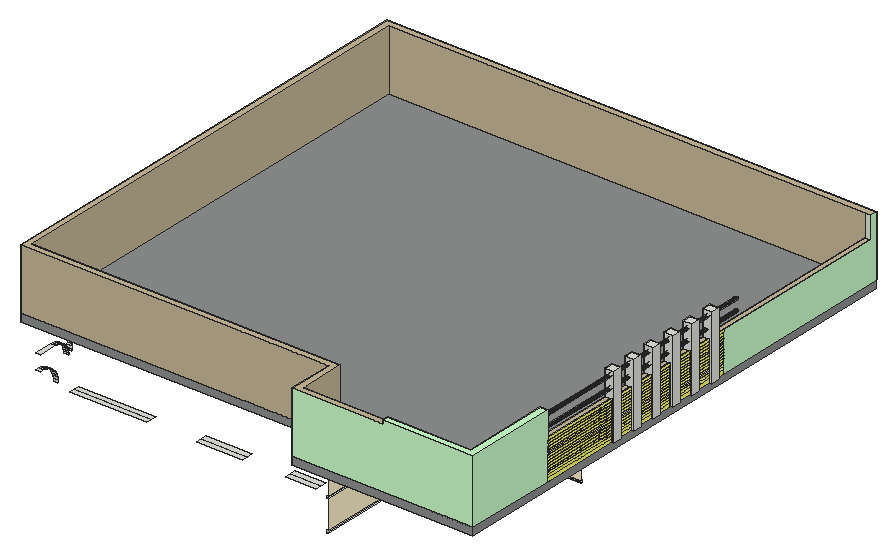
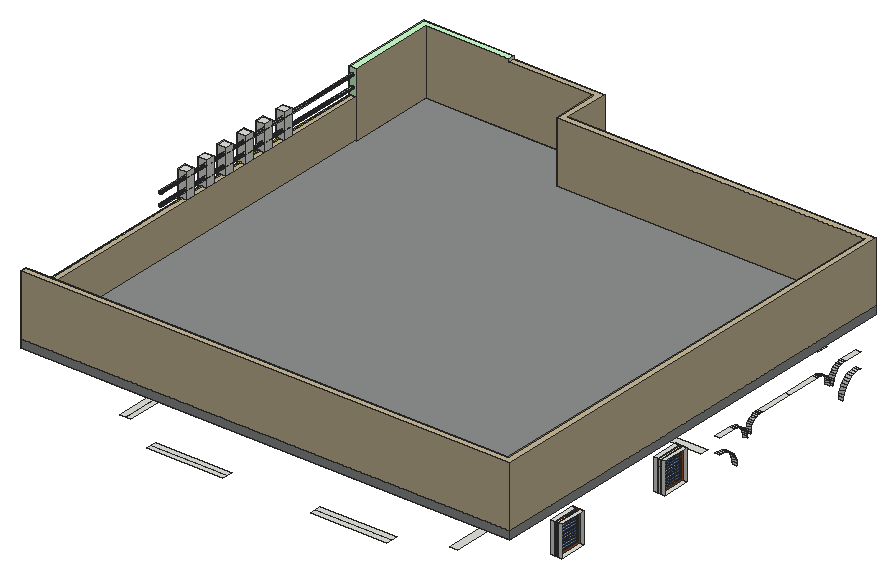
# SketchUp Ruby script. Lengths in inches.
U = 1.inch
M = Sketchup.active_model
def pt(a) = Geom::Point3d.new(a.map { |v| v * U })
def face(e, loops, mat)
  f = e.add_face(loops[0].map { |a| pt(a) })
  loops[1..].each { |l| e.add_face(l.map { |a| pt(a) }).erase! }
  f.material = f.back_material = mat if mat
  f
end
# faces: each face lists its corners as indices into pts; further lists are holes
def faces(e, pts, list, mat = nil) = list.each { |f| face(e, (f[0].is_a?(Array) ? f : [f]).map { |l| l.map { |i| pts[i] } }, mat) }
# xy, xz, yz: faces in a plane at the given z, y or x. An outline is a flat list of corners, or four numbers for a rectangle; further outlines are holes
def ring(l) = l.size == 4 ? [[l[0], l[1]], [l[2], l[1]], [l[2], l[3]], [l[0], l[3]]] : l.each_slice(2).to_a
def flat(e, list, mat, &to3) = list.each { |f| face(e, (f[0].is_a?(Array) ? f : [f]).map { |l| ring(l).map { |u, v| to3.(u, v) } }, mat) }
def xy(e, z, list, mat = nil) = flat(e, list, mat) { |x, y| [x, y, z] }
def xz(e, y, list, mat = nil) = flat(e, list, mat) { |x, z| [x, y, z] }
def yz(e, x, list, mat = nil) = flat(e, list, mat) { |y, z| [x, y, z] }
def lines(e, pts, list) = list.each { |a, b| e.add_line(pt(pts[a]), pt(pts[b])) }
# prism: a flat outline (further loops are holes) pulled along v
def prism(e, loops, v, mat = nil)
  f = face(e, loops, mat); d = Geom::Vector3d.new(v.map { |x| x * U })
  f.pushpull(f.normal.samedirection?(d) ? d.length : -d.length)
end
def box(e, o, s, mat = nil) = prism(e, [[o, [o[0] + s[0], o[1], o[2]], [o[0] + s[0], o[1] + s[1], o[2]], [o[0], o[1] + s[1], o[2]]]], [0, 0, s[2]], mat)
def at(x, y, z, deg = 0) = Geom::Transformation.translation(pt([x, y, z])) * Geom::Transformation.rotation(ORIGIN, Z_AXIS, deg.degrees)
def axes(o, x, y, z) = Geom::Transformation.new([*x, 0, *y, 0, *z, 0, *pt(o).to_a, 1])
def part(name) = M.definitions.add(name)
# library, detail: a bought-in or finely detailed component or shape, given as its bounding box
def library(name, o, s) = part(name).tap { |d| box(d.entities, o, s) }
def detail(e, o, s) = box(e.add_group.entities, o, s)
def put(e, d, t, mat = nil) = e.add_instance(d, t).tap { |i| i.material = mat if mat }
def group(e, t, mat = nil) = e.add_group.tap { |g| g.transformation = t; g.material = mat if mat }.entities
root = M.entities
M.materials.add("[Blacktop Old 02]").color = [143, 145, 145]
M.materials.add("[Color D01]").color = [255, 242, 204]
M.materials.add("[Color E03]").color = [255, 255, 101]
M.materials.add("[Color G01]").color = [204, 255, 204]
M.materials.add("[Metal Aluminum Anodized]").color = [202, 209, 219]
M.materials.add("[Quartz Light Brown]").color = [199, 184, 152]
M.materials.add("[Translucent Glass Blue]").color = [100, 149, 237]
M.materials["[Translucent Glass Blue]"].alpha = 0.5
M.materials.add("[Wood Cherry Original]").color = [152, 86, 42]
c1 = part("Group50\#1")
prism(c1.entities,[[[-9.82,-10.3125,0],[-9.82,-10.89,1],[-9.82,-9.89,1],[-9.82,-9.3125,0]]],[19.64,0,0])
c2 = part("Group51\#1")
prism(c2.entities,[[[-9.82,-7.89,1],[-9.82,-7.3125,0],[-9.82,-8.3125,0],[-9.82,-8.89,1]]],[19.64,0,0])
c3 = part("Group52\#1")
prism(c3.entities,[[[-9.82,-6.3125,0],[-9.82,-6.89,1],[-9.82,-5.89,1],[-9.82,-5.3125,0]]],[19.64,0,0])
c4 = part("Group53\#1")
prism(c4.entities,[[[9.82,-4.89,1],[9.82,-4.3125,0],[9.82,-3.3125,0],[9.82,-3.89,1]]],[-19.64,0,0])
c5 = part("Group54\#1")
prism(c5.entities,[[[-9.82,-1.89,1],[-9.82,-1.3125,0],[-9.82,-2.3125,0],[-9.82,-2.89,1]]],[19.64,0,0])
c6 = part("Group55\#1")
prism(c6.entities,[[[9.82,-0.3125,0],[9.82,0.6875,0],[9.82,0.11,1],[9.82,-0.89,1]]],[-19.64,0,0])
c7 = part("Group56\#1")
prism(c7.entities,[[[-9.82,2.11,1],[-9.82,2.6875,0],[-9.82,1.6875,0],[-9.82,1.11,1]]],[19.64,0,0])
c8 = part("Group57\#1")
prism(c8.entities,[[[-9.82,3.6875,0],[-9.82,3.11,1],[-9.82,4.11,1],[-9.82,4.6875,0]]],[19.64,0,0])
c9 = part("Group58\#1")
prism(c9.entities,[[[9.82,5.11,1],[9.82,5.6875,0],[9.82,6.6875,0],[9.82,6.11,1]]],[-19.64,0,0])
c10 = part("Group59\#1")
prism(c10.entities,[[[9.82,7.11,1],[9.82,7.6875,0],[9.82,8.6875,0],[9.82,8.11,1]]],[-19.64,0,0])
c11 = part("Group60\#1")
prism(c11.entities,[[[-9.82,9.6875,0],[-9.82,9.11,1],[-9.82,10.11,1],[-9.82,10.6875,0]]],[19.64,0,0])
c12 = part("Group48\#1")
put(c12.entities,c1,at(0,0,0),"[Translucent Glass Blue]")
put(c12.entities,c2,at(0,0,0),"[Translucent Glass Blue]")
put(c12.entities,c3,at(0,0,0),"[Translucent Glass Blue]")
put(c12.entities,c4,at(0,0,0),"[Translucent Glass Blue]")
put(c12.entities,c5,at(0,0,0),"[Translucent Glass Blue]")
put(c12.entities,c6,at(0,0,0),"[Translucent Glass Blue]")
put(c12.entities,c7,at(0,0,0),"[Translucent Glass Blue]")
put(c12.entities,c8,at(0,0,0),"[Translucent Glass Blue]")
put(c12.entities,c9,at(0,0,0),"[Translucent Glass Blue]")
put(c12.entities,c10,at(0,0,0),"[Translucent Glass Blue]")
put(c12.entities,c11,at(0,0,0),"[Translucent Glass Blue]")
c13 = part("Group62\#1")
prism(c13.entities,[[[9.56,-10.72,1],[9.56,-10.15,0],[9.56,-9.15,0],[9.56,-9.72,1]]],[-19.11,0,0])
c14 = part("Group63\#1")
prism(c14.entities,[[[-9.56,-7.15,0],[-9.56,-8.15,0],[-9.56,-8.72,1],[-9.56,-7.72,1]]],[19.11,0,0])
c15 = part("Group64\#1")
prism(c15.entities,[[[-9.56,-6.72,1],[-9.56,-5.72,1],[-9.56,-5.15,0],[-9.56,-6.15,0]]],[19.11,0,0])
c16 = part("Group65\#1")
prism(c16.entities,[[[9.56,-4.72,1],[9.56,-4.15,0],[9.56,-3.15,0],[9.56,-3.72,1]]],[-19.11,0,0])
c17 = part("Group66\#1")
prism(c17.entities,[[[-9.56,-2.72,1],[-9.56,-1.72,1],[-9.56,-1.15,0],[-9.56,-2.15,0]]],[19.11,0,0])
c18 = part("Group67\#1")
prism(c18.entities,[[[-9.56,-0.15,0],[-9.56,-0.72,1],[-9.56,0.28,1],[-9.56,0.85,0]]],[19.11,0,0])
c19 = part("Group68\#1")
prism(c19.entities,[[[-9.56,1.85,0],[-9.56,1.28,1],[-9.56,2.28,1],[-9.56,2.85,0]]],[19.11,0,0])
c20 = part("Group69\#1")
prism(c20.entities,[[[9.56,3.85,0],[9.56,4.85,0],[9.56,4.28,1],[9.56,3.28,1]]],[-19.11,0,0])
c21 = part("Group70\#1")
prism(c21.entities,[[[9.56,5.28,1],[9.56,5.85,0],[9.56,6.85,0],[9.56,6.28,1]]],[-19.11,0,0])
c22 = part("Group71\#1")
prism(c22.entities,[[[-9.56,8.85,0],[-9.56,7.85,0],[-9.56,7.28,1],[-9.56,8.28,1]]],[19.11,0,0])
c23 = part("Group72\#1")
xy(c23.entities,0,[[-9.56,9.85,9.56,10.72]])
xy(c23.entities,1,[[-9.56,9.28,9.56,10.28]])
p = [[9.56,9.28,1],[-9.56,9.28,1],[-9.56,9.85,0],[9.56,9.85,0],[-9.56,10.28,1],[9.56,10.28,1],
  [9.56,10.72,0.22],[-9.56,10.72,0.22]]
faces(c23.entities,p,[[0,1,2,3],[4,5,6,7]])
c24 = part("Group60\#2")
put(c24.entities,c13,at(0,0,0))
put(c24.entities,c14,at(0,0,0))
put(c24.entities,c15,at(0,0,0))
put(c24.entities,c16,at(0,0,0))
put(c24.entities,c17,at(0,0,0))
put(c24.entities,c18,at(0,0,0))
put(c24.entities,c19,at(0,0,0))
put(c24.entities,c20,at(0,0,0))
put(c24.entities,c21,at(0,0,0))
put(c24.entities,c22,at(0,0,0))
put(c24.entities,c23,at(0,0,0))
c25 = part("Group234\#2")
xy(c25.entities,126,[[595.96,-36,595.96,0,353.96,0,353.96,360,737.96,360,737.96,355,358.96,355,358.96,5,600.96,5,600.96,-31,666.96,-31,666.96,-36],[666.96,-36,732.27,-31],[732.27,-36,737.96,37.1875],[732.96,37.1875,737.96,355]])
xy(c25.entities,128.53,[[736.96,37.1875,737.96,210.375]])
xy(c25.entities,130.47,[[736.96,37.1875,737.96,210.375]])
xy(c25.entities,130.53,[[736.96,37.1875,737.96,210.375]])
xy(c25.entities,132.47,[[736.96,37.1875,737.96,210.375]])
xy(c25.entities,132.53,[[736.96,37.1875,737.96,210.375]])
xy(c25.entities,134.47,[[736.96,37.1875,737.96,210.375]])
xy(c25.entities,134.53,[[736.96,37.1875,737.96,210.375]])
xy(c25.entities,136.47,[[736.96,37.1875,737.96,210.375]])
xy(c25.entities,136.53,[[736.96,37.1875,737.96,210.375]])
xy(c25.entities,138.47,[[736.96,37.1875,737.96,210.375]])
xy(c25.entities,138.53,[[736.96,37.1875,737.96,210.375]])
xy(c25.entities,140.47,[[736.96,37.1875,737.96,210.375]])
xy(c25.entities,140.53,[[736.96,37.1875,737.96,210.375]])
xy(c25.entities,142.47,[[736.96,37.1875,737.96,210.375]])
xy(c25.entities,142.53,[[736.96,37.1875,737.96,210.375]])
xy(c25.entities,144.47,[[736.96,37.1875,737.96,210.375]])
xy(c25.entities,144.53,[[736.96,37.1875,737.96,210.375]])
xy(c25.entities,146.47,[[736.96,37.1875,737.96,210.375]])
xy(c25.entities,146.53,[[736.96,37.1875,737.96,210.375]])
xy(c25.entities,148.47,[[736.96,37.1875,737.96,210.375]])
xy(c25.entities,148.53,[[736.96,37.1875,737.96,210.375]])
xy(c25.entities,150.47,[[736.96,37.1875,737.96,210.375]])
xy(c25.entities,150.53,[[736.96,37.1875,737.96,210.375]])
xy(c25.entities,152.47,[[736.96,37.1875,737.96,210.375]])
xy(c25.entities,152.53,[[736.96,37.1875,737.96,210.375]])
xy(c25.entities,154.47,[[736.96,37.1875,737.96,210.375]])
xy(c25.entities,154.53,[[736.96,37.1875,737.96,210.375]])
xy(c25.entities,156.375,[[736.96,37.1875,737.96,355]],"[Color G01]")
xy(c25.entities,156.375,[[732.96,37.1875,736.96,355]],"[Quartz Light Brown]")
xy(c25.entities,174,[[595.96,-36,666.96,-36,666.96,-31,600.96,-31,600.96,5,358.96,5,358.96,355,737.96,355,737.96,360,353.96,360,353.96,0,595.96,0]],"[Quartz Light Brown]")
xy(c25.entities,176.4375,[[666.96,-36,737.96,-36,737.96,37.1875,732.27,37.1875,732.27,-31,666.96,-31]],"[Color G01]")
xz(c25.entities,-36,[[595.96,126,737.96,126,737.96,176.4375,666.96,176.4375,666.96,174,595.96,174]],"[Color G01]")
xz(c25.entities,-31,[[600.96,126,600.96,174,666.96,174,666.96,176.4375,732.27,176.4375,732.27,126]],"[Quartz Light Brown]")
xz(c25.entities,0,[[353.96,126,595.96,174]],"[Quartz Light Brown]")
xz(c25.entities,5,[[358.96,126,600.96,174]],"[Quartz Light Brown]")
xz(c25.entities,37.1875,[[732.96,126,732.96,156.375,736.96,156.375,736.96,154.53,737.96,154.53,737.96,154.47,736.96,154.47,736.96,152.53,737.96,152.53,737.96,152.47,736.96,152.47,736.96,150.53,737.96,150.53,737.96,150.47,736.96,150.47,736.96,148.53,737.96,148.53,737.96,148.47,736.96,148.47,736.96,146.53,737.96,146.53,737.96,146.47,736.96,146.47,736.96,144.53,737.96,144.53,737.96,144.47,736.96,144.47,736.96,142.53,737.96,142.53,737.96,142.47,736.96,142.47,736.96,140.53,737.96,140.53,737.96,140.47,736.96,140.47,736.96,138.53,737.96,138.53,737.96,138.47,736.96,138.47,736.96,136.53,737.96,136.53,737.96,136.47,736.96,136.47,736.96,134.53,737.96,134.53,737.96,134.47,736.96,134.47,736.96,132.53,737.96,132.53,737.96,132.47,736.96,132.47,736.96,130.53,737.96,130.53,737.96,130.47,736.96,130.47,736.96,128.53,737.96,128.53,737.96,126]])
xz(c25.entities,37.1875,[[732.27,126,732.27,176.4375,737.96,176.4375,737.96,156.375,732.96,156.375,732.96,126],[736.96,128.53,737.96,130.47],[736.96,130.53,737.96,132.47],[736.96,132.53,737.96,134.47],[736.96,134.53,737.96,136.47],
  [736.96,136.53,737.96,138.47],[736.96,138.53,737.96,140.47],[736.96,140.53,737.96,142.47],[736.96,142.53,737.96,144.47],[736.96,144.53,737.96,146.47],
  [736.96,146.53,737.96,148.47],[736.96,148.53,737.96,150.47],[736.96,150.53,737.96,152.47],[736.96,152.53,737.96,154.47],[736.96,154.53,737.96,156.375]],"[Color G01]")
xz(c25.entities,355,[[732.96,156.375,737.96,174]])
xz(c25.entities,355,[[358.96,126,732.96,174]],"[Quartz Light Brown]")
xz(c25.entities,360,[[353.96,126,737.96,174]],"[Quartz Light Brown]")
yz(c25.entities,353.96,[[0,126,360,174]],"[Quartz Light Brown]")
yz(c25.entities,358.96,[[5,126,355,174]],"[Quartz Light Brown]")
yz(c25.entities,595.96,[[-36,126,0,174]],"[Quartz Light Brown]")
yz(c25.entities,600.96,[[-31,126,5,174]],"[Quartz Light Brown]")
yz(c25.entities,666.96,[[-36,174,-31,176.4375]])
yz(c25.entities,732.27,[[-31,126,37.1875,176.4375]],"[Quartz Light Brown]")
yz(c25.entities,732.96,[[37.1875,126,355,156.375]],"[Quartz Light Brown]")
yz(c25.entities,736.96,[[37.1875,128.53,210.375,130.47],[37.1875,130.53,210.375,132.47],[37.1875,132.53,210.375,134.47],[37.1875,134.53,210.375,136.47],[37.1875,136.53,210.375,138.47],
  [37.1875,138.53,210.375,140.47],[37.1875,140.53,210.375,142.47],[37.1875,142.53,210.375,144.47],[37.1875,144.53,210.375,146.47],[37.1875,146.53,210.375,148.47],
  [37.1875,148.53,210.375,150.47],[37.1875,150.53,210.375,152.47],[37.1875,152.53,210.375,154.47],[37.1875,154.53,210.375,156.375]],"[Color E03]")
yz(c25.entities,737.96,[[100.3125,128.53,106.95,130.47],[37.1875,130.47,90.98,130.53],[90.98,130.47,94.56,130.53],[94.56,130.47,100.3125,130.53],[100.3125,130.47,106.95,130.53],
  [106.95,130.47,210.375,130.53],[100.3125,130.53,106.95,132.47],[37.1875,132.47,90.98,132.53],[90.98,132.47,94.56,132.53],[94.56,132.47,100.3125,132.53],
  [100.3125,132.47,106.95,132.53],[106.95,132.47,210.375,132.53],[100.3125,132.53,106.95,134.47],[37.1875,134.47,90.98,134.53],[90.98,134.47,94.56,134.53],
  [94.56,134.47,100.3125,134.53],[100.3125,134.47,106.95,134.53],[106.95,134.47,210.375,134.53],[100.3125,134.53,106.95,136.47],[37.1875,136.47,90.98,136.53],
  [90.98,136.47,94.56,136.53],[94.56,136.47,100.3125,136.53],[100.3125,136.47,106.95,136.53],[106.95,136.47,210.375,136.53],[100.3125,136.53,106.95,138.47],
  [37.1875,138.47,90.98,138.53],[90.98,138.47,94.56,138.53],[94.56,138.47,100.3125,138.53],[100.3125,138.47,106.95,138.53],[106.95,138.47,210.375,138.53],
  [100.3125,138.53,106.95,140.47],[37.1875,140.47,90.98,140.53],[90.98,140.47,94.56,140.53],[94.56,140.47,100.3125,140.53],[100.3125,140.47,106.95,140.53],
  [106.95,140.47,210.375,140.53],[100.3125,140.53,106.95,142.47],[37.1875,142.47,90.98,142.53],[90.98,142.47,94.56,142.53],[94.56,142.47,100.3125,142.53],
  [100.3125,142.47,106.95,142.53],[106.95,142.47,210.375,142.53],[100.3125,142.53,106.95,144.47],[37.1875,144.47,90.98,144.53],[90.98,144.47,94.56,144.53],
  [94.56,144.47,100.3125,144.53],[100.3125,144.47,106.95,144.53],[106.95,144.47,210.375,144.53],[100.3125,144.53,106.95,146.47],[37.1875,146.47,90.98,146.53],
  [90.98,146.47,94.56,146.53],[94.56,146.47,100.3125,146.53],[100.3125,146.47,106.95,146.53],[106.95,146.47,210.375,146.53],[100.3125,146.53,106.95,148.47],
  [37.1875,148.47,90.98,148.53],[90.98,148.47,94.56,148.53],[94.56,148.47,100.3125,148.53],[100.3125,148.47,106.95,148.53],[106.95,148.47,210.375,148.53],
  [100.3125,148.53,106.95,150.47],[37.1875,150.47,90.98,150.53],[90.98,150.47,94.56,150.53],[94.56,150.47,100.3125,150.53],[100.3125,150.47,106.95,150.53],
  [106.95,150.47,210.375,150.53],[100.3125,150.53,106.95,152.47],[37.1875,152.47,90.98,152.53],[90.98,152.47,94.56,152.53],[94.56,152.47,100.3125,152.53],
  [100.3125,152.47,106.95,152.53],[106.95,152.47,210.375,152.53],[100.3125,152.53,106.95,154.47],[37.1875,154.47,90.98,154.53],[90.98,154.47,94.56,154.53],
  [94.56,154.47,100.3125,154.53],[100.3125,154.47,106.95,154.53],[106.95,154.47,210.375,154.53]])
yz(c25.entities,737.96,[[37.1875,126,100.3125,128.53],[100.3125,126,106.95,128.53],[106.95,126,210.375,128.53],[37.1875,128.53,100.3125,130.47],[106.95,128.53,210.375,130.47],
  [37.1875,130.53,100.3125,132.47],[106.95,130.53,210.375,132.47],[37.1875,132.53,100.3125,134.47],[106.95,132.53,210.375,134.47],[37.1875,134.53,100.3125,136.47],
  [106.95,134.53,210.375,136.47],[37.1875,136.53,100.3125,138.47],[106.95,136.53,210.375,138.47],[37.1875,138.53,100.3125,140.47],[106.95,138.53,210.375,140.47],
  [37.1875,140.53,100.3125,142.47],[106.95,140.53,210.375,142.47],[37.1875,142.53,100.3125,144.47],[106.95,142.53,210.375,144.47],[37.1875,144.53,100.3125,146.47],
  [106.95,144.53,210.375,146.47],[37.1875,146.53,100.3125,148.47],[106.95,146.53,210.375,148.47],[37.1875,148.53,100.3125,150.47],[106.95,148.53,210.375,150.47],
  [37.1875,150.53,100.3125,152.47],[106.95,150.53,210.375,152.47],[37.1875,152.53,100.3125,154.47],[106.95,152.53,210.375,154.47],[37.1875,154.53,100.3125,156.375],
  [106.95,154.53,210.375,156.375]],"[Color E03]")
yz(c25.entities,737.96,[[-36,126,37.1875,176.4375],[210.375,126,360,126,360,174,355,174,355,156.375,210.375,156.375]],"[Color G01]")
g1 = group(c25.entities,at(737.96,100.3125,154.53))
xy(g1,-28.53,[[0,0,2,6.64]])
xy(g1,1.84,[[-5,0,0,6.64]])
xy(g1,21.9,[[-5,0,2,6.64]])
xz(g1,0,[[0,-28.53,2,-28.53,2,21.9,-5,21.9,-5,1.84,0,1.84]])
xz(g1,6.64,[[0,-28.53,2,1.84],[-5,1.84,2,21.9]])
yz(g1,-5,[[0,1.84,6.64,21.9]])
yz(g1,0,[[0,-28.53,6.64,1.84]])
yz(g1,2,[[0,-28.53,6.64,21.9]])
g2 = group(c25.entities,at(737.96,119.4375,154.53))
xy(g2,-28.53,[[0,0,2,6.64]])
xy(g2,1.84,[[-5,0,0,6.64]])
xy(g2,21.9,[[-5,0,2,6.64]])
xz(g2,0,[[0,-28.53,2,-28.53,2,21.9,-5,21.9,-5,1.84,0,1.84]])
xz(g2,6.64,[[0,-28.53,2,1.84],[-5,1.84,2,21.9]])
yz(g2,-5,[[0,1.84,6.64,21.9]])
yz(g2,0,[[0,-28.53,6.64,1.84]])
yz(g2,2,[[0,-28.53,6.64,21.9]])
g3 = group(c25.entities,at(737.96,138.5625,154.53))
xy(g3,-28.53,[[0,0,2,6.64]])
xy(g3,1.84,[[-5,0,0,6.64]])
xy(g3,21.9,[[-5,0,2,6.64]])
xz(g3,0,[[0,-28.53,2,-28.53,2,21.9,-5,21.9,-5,1.84,0,1.84]])
xz(g3,6.64,[[0,-28.53,2,1.84],[-5,1.84,2,21.9]])
yz(g3,-5,[[0,1.84,6.64,21.9]])
yz(g3,0,[[0,-28.53,6.64,1.84]])
yz(g3,2,[[0,-28.53,6.64,21.9]])
g4 = group(c25.entities,at(737.96,157.6875,154.53))
xy(g4,-28.53,[[0,0,2,6.64]])
xy(g4,1.84,[[-5,0,0,6.64]])
xy(g4,21.9,[[-5,0,2,6.64]])
xz(g4,0,[[0,-28.53,2,-28.53,2,21.9,-5,21.9,-5,1.84,0,1.84]])
xz(g4,6.64,[[0,-28.53,2,1.84],[-5,1.84,2,21.9]])
yz(g4,-5,[[0,1.84,6.64,21.9]])
yz(g4,0,[[0,-28.53,6.64,1.84]])
yz(g4,2,[[0,-28.53,6.64,21.9]])
g5 = group(c25.entities,at(737.96,176.8125,154.53))
xy(g5,-28.53,[[0,0,2,6.64]])
xy(g5,1.84,[[-5,0,0,6.64]])
xy(g5,21.72,[[-5,0,2,6.64]])
xz(g5,0,[[0,-28.53,2,-28.53,2,21.72,-5,21.72,-5,1.84,0,1.84]])
xz(g5,6.64,[[0,-28.53,2,1.84],[-5,1.84,2,21.72]])
yz(g5,-5,[[0,1.84,6.64,21.72]])
yz(g5,0,[[0,-28.53,6.64,1.84]])
yz(g5,2,[[0,-28.53,6.64,21.72]])
g6 = group(c25.entities,at(737.96,195.9375,154.53))
xy(g6,-28.53,[[0,0,2,6.64]])
xy(g6,1.84,[[-5,0,0,6.64]])
xy(g6,21.72,[[-5,0,2,6.64]])
xz(g6,0,[[0,-28.53,2,-28.53,2,21.72,-5,21.72,-5,1.84,0,1.84]])
xz(g6,6.64,[[0,-28.53,2,1.84],[-5,1.84,2,21.72]])
yz(g6,-5,[[0,1.84,6.64,21.72]])
yz(g6,0,[[0,-28.53,6.64,1.84]])
yz(g6,2,[[0,-28.53,6.64,21.72]])
xy(root,56.32,[[241,36,242,133.9],[241,169.9,242,169.9,242,181,241,182],[242,181,324,181,324,182,241,182]])
xy(root,58.26,[[241,36,242,133.9],[241,169.9,241,182,242,181,242,169.9],[242,181,241,182,324,182,324,181]])
xy(root,80.32,[[241,36,242,133.9],[241,169.9,242,169.9,242,181,241,182],[242,181,324,181,324,182,241,182]])
xy(root,82.26,[[241,36,242,133.9],[241,169.9,241,182,242,181,242,169.9],[242,181,241,182,324,182,324,181]])
xy(root,84,[[39,36,99,45],[138.68,36,174.68,45],[208.27,36,232.27,45],[236.5,133.9,242,169.9],[129,140.13,134.5,176.13],
  [15,183,51,189],[315,199.85,324,259.85],[0,221.625,9,243.48],[3.5,221.625,5.5,243.48],[189,274.07,195,310.07],
  [315,313.375,324,373.375],[0,322.71,3.5,344.375],[3.5,322.71,4.5,344.375],[4.5,322.71,5.5,344.375],[5.5,322.71,9,344.375],
  [57,339.41,63,375.41],[96,387,156,396],[225,387,285,396]])
xy(root,85.11,[[3.5,222.74,4.5,242.37],[4.5,222.74,5.5,242.37]],"[Wood Cherry Original]")
xy(root,85.28,[[3.5,323.98,5.5,343.1]],"[Wood Cherry Original]")
xy(root,95.9375,[[5.25,87,9,114],[5.25,114,9,141]])
xy(root,96,[[5.25,45,9,59.65],[5.25,168.35,9,183]])
xy(root,104.32,[[241,36,242,36,242,181,241,182],[242,181,324,181,324,182,241,182]])
xy(root,106.26,[[241,36,241,182,242,181,242,36],[242,181,241,182,324,182,324,181]])
xy(root,106.72,[[3.5,323.98,5.5,343.1]])
xy(root,106.89,[[3.5,222.74,5.5,242.37]],"[Wood Cherry Original]")
xy(root,108,[[0,221.625,9,243.48],[3.5,221.625,5.5,243.48],[0,322.71,3.5,344.375],[3.5,322.71,4.5,344.375],[4.5,322.71,5.5,344.375],
  [5.5,322.71,9,344.375]])
xy(root,120,[[[0,36,242,36,242,181,324,181,324,396,0,396],[134.5,45,134.5,189,63,189,63,261,202.86,261,202.86,267,195,267,195,387,315,387,315,190,236.5,190,236.5,111.96,193.6875,111.96,193.6875,105.96,236.5,105.96,236.5,45],[9,45,129,183],[63,267,189,387],[9,267,57,387],[9,189,57,261]]])
xz(root,73.1875,[[381.31,161.17,381.59,161.2,381.84,161.31,382.0625,161.48,382.23,161.7,382.34,161.96,382.375,162.23,382.34,162.51,382.23,162.76,382.0625,162.99,381.84,163.15,381.59,163.26,381.31,163.3,381.03,163.26,380.78,163.15,380.56,162.99,380.39,162.76,380.28,162.51,380.24,162.23,380.28,161.96,380.39,161.7,380.56,161.48,380.78,161.31,381.03,161.2]])
xz(root,73.1875,[[381.31,170.15,381.59,170.19,381.84,170.29,382.0625,170.46,382.23,170.68,382.34,170.9375,382.375,171.21,382.34,171.49,382.23,171.75,382.0625,171.97,381.84,172.14,381.59,172.24,381.31,172.28,381.03,172.24,380.78,172.14,380.56,171.97,380.39,171.75,380.28,171.49,380.24,171.21,380.28,170.9375,380.39,170.68,380.56,170.46,380.78,170.29,381.03,170.19]],"[Metal Aluminum Anodized]")
xz(root,133.9,[[241,56.32,242,58.26],[241,80.32,242,82.26]])
xz(root,169.9,[[241,56.32,242,58.26],[241,80.32,242,82.26]])
xz(root,181,[[242,58.26,324,80.32],[242,82.26,324,104.32],[242,106.26,324,120]],"[Color D01]")
xz(root,182,[[241,56.32,324,58.26],[241,80.32,324,82.26],[241,104.32,324,106.26]])
xz(root,221.625,[[0,84,9,108],[3.5,84,5.5,108]])
xz(root,222.74,[[3.5,85.11,4.5,106.89],[4.5,85.11,5.5,106.89]],"[Wood Cherry Original]")
xz(root,242.37,[[3.5,85.11,4.5,106.89],[4.5,85.11,5.5,106.89]],"[Wood Cherry Original]")
xz(root,243.48,[[0,84,9,108],[3.5,84,5.5,108]])
xz(root,262.0625,[[381.31,161.17,381.03,161.2,380.78,161.31,380.56,161.48,380.39,161.7,380.28,161.96,380.24,162.23,380.28,162.51,380.39,162.76,380.56,162.99,380.78,163.15,381.03,163.26,381.31,163.3,381.59,163.26,381.84,163.15,382.0625,162.99,382.23,162.76,382.34,162.51,382.375,162.23,382.34,161.96,382.23,161.7,382.0625,161.48,381.84,161.31,381.59,161.2]])
xz(root,262.0625,[[381.31,170.15,381.03,170.19,380.78,170.29,380.56,170.46,380.39,170.68,380.28,170.9375,380.24,171.21,380.28,171.49,380.39,171.75,380.56,171.97,380.78,172.14,381.03,172.24,381.31,172.28,381.59,172.24,381.84,172.14,382.0625,171.97,382.23,171.75,382.34,171.49,382.375,171.21,382.34,170.9375,382.23,170.68,382.0625,170.46,381.84,170.29,381.59,170.19]],"[Metal Aluminum Anodized]")
xz(root,322.71,[[0,84,3.5,108],[3.5,84,4.5,108],[4.5,84,5.5,108],[5.5,84,9,108]])
xz(root,323.98,[[3.5,85.28,5.5,106.72]],"[Wood Cherry Original]")
xz(root,343.1,[[3.5,85.28,5.5,106.72]],"[Wood Cherry Original]")
xz(root,344.375,[[0,84,3.5,108],[3.5,84,4.5,108],[4.5,84,5.5,108],[5.5,84,9,108]])
yz(root,3.5,[[[221.625,84,243.48,108],[222.74,85.11,242.37,106.89]],[[322.71,84,344.375,108],[323.98,85.28,343.1,106.72]]],"[Wood Cherry Original]")
yz(root,5.5,[[[221.625,84,243.48,108],[222.74,85.11,242.37,106.89]],[[322.71,84,344.375,108],[323.98,85.28,343.1,106.72]]],"[Wood Cherry Original]")
yz(root,241,[[36,56.32,133.9,58.26],[169.9,56.32,182,58.26],[36,80.32,133.9,82.26],[169.9,80.32,182,82.26],[36,104.32,182,106.26]])
yz(root,242,[[36,58.26,133.9,80.32],[169.9,58.26,181,80.32],[36,82.26,133.9,82.26,133.9,84,169.9,84,169.9,82.26,181,82.26,181,104.32,36,104.32],[36,106.26,181,120]],"[Color D01]")
p = [[9,61.85,71.03],[9,62,68.89],[5.25,62,68.89],[5.25,61.85,71.03],[9,166,68.89],[9,166.15,71.03],
  [5.25,166.15,71.03],[5.25,166,68.89],[9,61.4,73.12],[5.25,61.4,73.12],[9,166.6,73.12],[5.25,166.6,73.12],
  [9,60.66,75.125],[5.25,60.66,75.125],[9,167.34,75.125],[5.25,167.34,75.125],[9,59.65,77.01],[5.25,59.65,77.01],
  [9,168.35,77.01],[5.25,168.35,77.01],[9,58.39,78.74],[5.25,58.39,78.74],[9,169.61,78.74],[5.25,169.61,78.74],
  [9,56.89,80.26],[5.25,56.89,80.26],[9,171.11,80.26],[5.25,171.11,80.26],[9,55.2,81.57],[5.25,55.2,81.57],
  [9,172.8,81.57],[5.25,172.8,81.57],[9,53.34,82.625],[5.25,53.34,82.625],[9,174.66,82.625],[5.25,174.66,82.625],
  [9,51.35,83.41],[5.25,51.35,83.41],[9,176.65,83.41],[5.25,176.65,83.41],[9,49.27,83.9],[5.25,49.27,83.9],
  [9,178.73,83.9],[5.25,178.73,83.9],[9,47.14,84.1],[5.25,47.14,84.1],[9,180.86,84.1],[5.25,180.86,84.1],
  [9,45,84],[5.25,45,84],[9,72,84],[9,71.89,85.6],[5.25,71.89,85.6],[5.25,72,84],
  [9,156.11,85.6],[9,156,84],[5.25,156,84],[5.25,156.11,85.6],[9,183,84],[5.25,183,84],
  [9,71.58,87.16],[5.25,71.58,87.16],[9,75.03,87.12],[9,75,85.6],[5.25,75,85.6],[5.25,75.03,87.12],
  [9,153,85.6],[9,152.97,87.12],[5.25,152.97,87.12],[5.25,153,85.6],[9,156.42,87.16],[5.25,156.42,87.16],
  [9,75.29,88.62],[5.25,75.29,88.62],[9,152.71,88.62],[5.25,152.71,88.62],[9,71.05,88.67],[5.25,71.05,88.67],
  [9,156.95,88.67],[5.25,156.95,88.67],[9,75.77,90.07],[5.25,75.77,90.07],[9,152.23,90.07],[5.25,152.23,90.07],
  [9,70.33,90.1],[5.25,70.33,90.1],[9,157.67,90.1],[5.25,157.67,90.1],[9,69.43,91.42],[5.25,69.43,91.42],
  [9,76.47,91.42],[5.25,76.47,91.42],[9,151.53,91.42],[5.25,151.53,91.42],[9,158.57,91.42],[5.25,158.57,91.42],
  [9,68.36,92.61],[5.25,68.36,92.61],[9,77.37,92.65],[5.25,77.37,92.65],[9,150.63,92.65],[5.25,150.63,92.65],
  [9,159.64,92.61],[5.25,159.64,92.61],[9,67.14,93.64],[5.25,67.14,93.64],[9,160.86,93.64],[5.25,160.86,93.64],
  [9,78.44,93.73],[5.25,78.44,93.73],[9,149.56,93.73],[5.25,149.56,93.73],[9,65.8,94.51],[5.25,65.8,94.51],
  [9,162.2,94.51],[5.25,162.2,94.51],[9,79.67,94.64],[5.25,79.67,94.64],[9,148.33,94.64],[5.25,148.33,94.64],
  [9,64.35,95.1875],[5.25,64.35,95.1875],[9,163.65,95.1875],[5.25,163.65,95.1875],[9,81.02,95.34],[5.25,81.02,95.34],
  [9,146.98,95.34],[5.25,146.98,95.34],[9,62.83,95.67],[5.25,62.83,95.67],[9,165.17,95.67],[5.25,165.17,95.67],
  [9,82.46,95.84],[5.25,82.46,95.84],[9,145.54,95.84],[5.25,145.54,95.84],[9,61.25,95.9375],[5.25,61.25,95.9375],
  [9,166.75,95.9375],[5.25,166.75,95.9375],[9,83.96,96.1],[5.25,83.96,96.1],[9,144.04,96.1],[5.25,144.04,96.1],
  [9,59.65,96],[5.25,59.65,96],[9,87,95.9375],[9,85.49,96.14],[5.25,85.49,96.14],[5.25,87,95.9375],
  [9,142.51,96.14],[9,141,95.9375],[5.25,141,95.9375],[5.25,142.51,96.14],[9,168.35,96],[5.25,168.35,96],
  [381.03,73.1875,161.2],[380.78,73.1875,161.31],[380.78,136.3125,161.31],[380.78,262.0625,161.31],[381.03,262.0625,161.2],[381.03,136.3125,161.2],
  [381.31,73.1875,161.17],[381.31,262.0625,161.17],[381.31,136.3125,161.17],[381.59,73.1875,161.2],[381.59,262.0625,161.2],[381.59,136.3125,161.2],
  [381.84,262.0625,161.31],[381.84,136.3125,161.31],[381.84,73.1875,161.31],[380.56,136.3125,161.48],[380.56,262.0625,161.48],[380.56,73.1875,161.48],
  [382.0625,262.0625,161.48],[382.0625,136.3125,161.48],[382.0625,73.1875,161.48],[380.39,136.3125,161.7],[380.39,262.0625,161.7],[380.39,73.1875,161.7],
  [382.23,262.0625,161.7],[382.23,136.3125,161.7],[382.23,73.1875,161.7],[380.28,136.3125,161.96],[380.28,262.0625,161.96],[380.28,73.1875,161.96],
  [382.34,262.0625,161.96],[382.34,136.3125,161.96],[382.34,73.1875,161.96],[380.24,136.3125,162.23],[380.24,262.0625,162.23],[380.24,73.1875,162.23],
  [382.375,262.0625,162.23],[382.375,136.3125,162.23],[382.375,73.1875,162.23],[380.28,136.3125,162.51],[380.28,262.0625,162.51],[380.28,73.1875,162.51],
  [382.34,262.0625,162.51],[382.34,136.3125,162.51],[382.34,73.1875,162.51],[380.39,136.3125,162.76],[380.39,262.0625,162.76],[380.39,73.1875,162.76],
  [382.23,262.0625,162.76],[382.23,136.3125,162.76],[382.23,73.1875,162.76],[380.56,136.3125,162.99],[380.56,262.0625,162.99],[380.56,73.1875,162.99],
  [382.0625,262.0625,162.99],[382.0625,136.3125,162.99],[382.0625,73.1875,162.99],[380.78,136.3125,163.15],[380.78,262.0625,163.15],[380.78,73.1875,163.15],
  [381.84,262.0625,163.15],[381.84,136.3125,163.15],[381.84,73.1875,163.15],[381.03,136.3125,163.26],[381.03,262.0625,163.26],[381.03,73.1875,163.26],
  [381.59,262.0625,163.26],[381.59,136.3125,163.26],[381.59,73.1875,163.26],[381.31,136.3125,163.3],[381.31,262.0625,163.3],[381.31,73.1875,163.3],
  [381.31,73.1875,170.15],[381.03,73.1875,170.19],[381.03,136.3125,170.19],[381.03,262.0625,170.19],[381.31,262.0625,170.15],[381.31,136.3125,170.15],
  [381.59,73.1875,170.19],[381.59,262.0625,170.19],[381.59,136.3125,170.19],[380.78,73.1875,170.29],[380.78,136.3125,170.29],[380.78,262.0625,170.29],
  [381.84,262.0625,170.29],[381.84,136.3125,170.29],[381.84,73.1875,170.29],[380.56,136.3125,170.46],[380.56,262.0625,170.46],[380.56,73.1875,170.46],
  [382.0625,262.0625,170.46],[382.0625,136.3125,170.46],[382.0625,73.1875,170.46],[380.39,136.3125,170.68],[380.39,262.0625,170.68],[380.39,73.1875,170.68],
  [382.23,262.0625,170.68],[382.23,136.3125,170.68],[382.23,73.1875,170.68],[380.28,136.3125,170.9375],[380.28,262.0625,170.9375],[380.28,73.1875,170.9375],
  [382.34,262.0625,170.9375],[382.34,136.3125,170.9375],[382.34,73.1875,170.9375],[380.24,136.3125,171.21],[380.24,262.0625,171.21],[380.24,73.1875,171.21],
  [382.375,262.0625,171.21],[382.375,136.3125,171.21],[382.375,73.1875,171.21],[380.28,136.3125,171.49],[380.28,262.0625,171.49],[380.28,73.1875,171.49],
  [382.34,262.0625,171.49],[382.34,136.3125,171.49],[382.34,73.1875,171.49],[380.39,136.3125,171.75],[380.39,262.0625,171.75],[380.39,73.1875,171.75],
  [382.23,262.0625,171.75],[382.23,136.3125,171.75],[382.23,73.1875,171.75],[380.56,136.3125,171.97],[380.56,262.0625,171.97],[380.56,73.1875,171.97],
  [382.0625,262.0625,171.97],[382.0625,136.3125,171.97],[382.0625,73.1875,171.97],[380.78,136.3125,172.14],[380.78,262.0625,172.14],[380.78,73.1875,172.14],
  [381.84,262.0625,172.14],[381.84,136.3125,172.14],[381.84,73.1875,172.14],[381.03,136.3125,172.24],[381.03,262.0625,172.24],[381.03,73.1875,172.24],
  [381.59,262.0625,172.24],[381.59,136.3125,172.24],[381.59,73.1875,172.24],[381.31,136.3125,172.28],[381.31,262.0625,172.28],[381.31,73.1875,172.28],
  [39,40.5,84],[99,40.5,84],[138.68,40.5,84],[174.68,40.5,84],[208.27,40.5,84],[232.27,40.5,84],
  [319.5,259.85,84],[319.5,199.85,84],[319.5,373.375,84],[319.5,313.375,84],[285,391.5,84],[225,391.5,84],
  [156,391.5,84],[96,391.5,84],[4.5,323.98,106.72],[4.5,343.1,106.72],[4.5,343.1,85.28],[4.5,323.98,85.28],
  [381.31,73.1875,171.21],[381.31,136.3125,171.21],[381.31,262.0625,171.21]]
faces(root,p,[[0,1,2,3],[4,5,6,7],[8,0,3,9],[5,10,11,6],[12,8,9,13],[10,14,15,11],[16,12,13,17],[14,18,19,15],
  [20,16,17,21],[18,22,23,19],[24,20,21,25],[22,26,27,23],[28,24,25,29],[26,30,31,27],[32,28,29,33],[30,34,35,31],
  [36,32,33,37],[34,38,39,35],[40,36,37,41],[38,42,43,39],[44,40,41,45],[42,46,47,43],[48,44,45,49],[50,51,52,53],
  [54,55,56,57],[46,58,59,47],[51,60,61,52],[62,63,64,65],[66,67,68,69],[70,54,57,71],[72,62,65,73],[67,74,75,68],
  [60,76,77,61],[78,70,71,79],[80,72,73,81],[74,82,83,75],[76,84,85,77],[86,78,79,87],[84,88,89,85],[90,80,81,91],
  [82,92,93,83],[94,86,87,95],[88,96,97,89],[98,90,91,99],[92,100,101,93],[102,94,95,103],[96,104,105,97],[106,102,103,107],
  [108,98,99,109],[100,110,111,101],[104,112,113,105],[114,106,107,115],[116,108,109,117],[110,118,119,111],[112,120,121,113],[122,114,115,123],
  [124,116,117,125],[118,126,127,119],[120,128,129,121],[130,122,123,131],[132,124,125,133],[126,134,135,127],[128,136,137,129],[138,130,131,139],
  [140,132,133,141],[134,142,143,135],[136,144,145,137],[146,147,148,149],[150,151,152,153],[154,138,139,155],[147,140,141,148],[142,150,153,143]])
faces(root,p,[[156,157,158,159,160,161],[162,156,161,160,163,164],[165,162,164,163,166,167],[167,166,168,169,170,165],[171,172,159,158,157,173],[169,168,174,175,176,170],[177,178,172,171,173,179],[175,174,180,181,182,176],
  [183,184,178,177,179,185],[181,180,186,187,188,182],[189,190,184,183,185,191],[187,186,192,193,194,188],[195,196,190,189,191,197],[193,192,198,199,200,194],[201,202,196,195,197,203],[199,198,204,205,206,200],
  [207,208,202,201,203,209],[205,204,210,211,212,206],[213,214,208,207,209,215],[211,210,216,217,218,212],[219,220,214,213,215,221],[217,216,222,223,224,218],[225,226,220,219,221,227],[223,222,226,225,227,224],
  [228,229,230,231,232,233],[234,228,233,232,235,236],[229,237,238,239,231,230],[236,235,240,241,242,234],[243,244,239,238,237,245],[241,240,246,247,248,242],[249,250,244,243,245,251],[247,246,252,253,254,248],
  [255,256,250,249,251,257],[253,252,258,259,260,254],[261,262,256,255,257,263],[259,258,264,265,266,260],[267,268,262,261,263,269],[265,264,270,271,272,266],[273,274,268,267,269,275],[271,270,276,277,278,272],
  [279,280,274,273,275,281],[277,276,282,283,284,278],[285,286,280,279,281,287],[283,282,288,289,290,284],[291,292,286,285,287,293],[289,288,294,295,296,290],[297,298,292,291,293,299],[295,294,298,297,299,296]],"[Metal Aluminum Anodized]")
lines(root,p,[[300,301],[302,303],[304,305],[306,307],[308,309],[310,311],[312,313],[314,315],[315,316],[316,317],[317,314],[318,319],
  [319,320]])
put(root,c12,axes([5,232.55,96],[0,-1,0],[0,0,1],[-1,0,0]))
put(root,c24,axes([5,333.54,96],[0,-1,0],[0,0,1],[-1,0,0]),"[Translucent Glass Blue]")
g7 = group(root,at(0,36,120),"[Blacktop Old 02]")
prism(g7,[[[0,0,0],[0,360,0],[384,360,0],[384,-36,0],[242,-36,0],[242,0,0]]],[0,0,6])
put(root,c25,at(-353.96,36,0))
